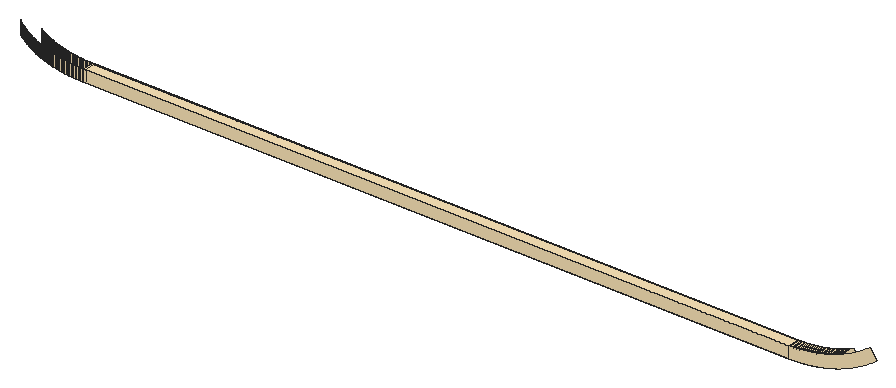
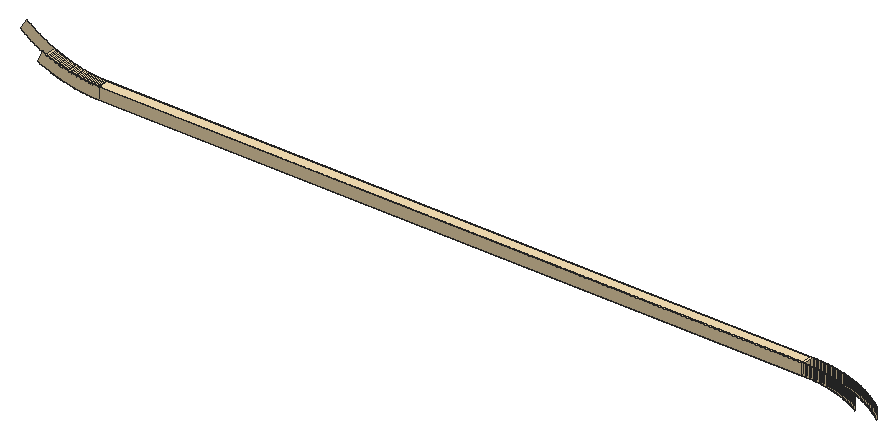
# SketchUp Ruby script. Lengths in inches.
U = 1.inch
M = Sketchup.active_model
def pt(a) = Geom::Point3d.new(a.map { |v| v * U })
def face(e, loops, mat)
  f = e.add_face(loops[0].map { |a| pt(a) })
  loops[1..].each { |l| e.add_face(l.map { |a| pt(a) }).erase! }
  f.material = f.back_material = mat if mat
  f
end
# faces: each face lists its corners as indices into pts; further lists are holes
def faces(e, pts, list, mat = nil) = list.each { |f| face(e, (f[0].is_a?(Array) ? f : [f]).map { |l| l.map { |i| pts[i] } }, mat) }
# xy, xz, yz: faces in a plane at the given z, y or x. An outline is a flat list of corners, or four numbers for a rectangle; further outlines are holes
def ring(l) = l.size == 4 ? [[l[0], l[1]], [l[2], l[1]], [l[2], l[3]], [l[0], l[3]]] : l.each_slice(2).to_a
def flat(e, list, mat, &to3) = list.each { |f| face(e, (f[0].is_a?(Array) ? f : [f]).map { |l| ring(l).map { |u, v| to3.(u, v) } }, mat) }
def xy(e, z, list, mat = nil) = flat(e, list, mat) { |x, y| [x, y, z] }
def xz(e, y, list, mat = nil) = flat(e, list, mat) { |x, z| [x, y, z] }
def yz(e, x, list, mat = nil) = flat(e, list, mat) { |y, z| [x, y, z] }
def lines(e, pts, list) = list.each { |a, b| e.add_line(pt(pts[a]), pt(pts[b])) }
# prism: a flat outline (further loops are holes) pulled along v
def prism(e, loops, v, mat = nil)
  f = face(e, loops, mat); d = Geom::Vector3d.new(v.map { |x| x * U })
  f.pushpull(f.normal.samedirection?(d) ? d.length : -d.length)
end
def box(e, o, s, mat = nil) = prism(e, [[o, [o[0] + s[0], o[1], o[2]], [o[0] + s[0], o[1] + s[1], o[2]], [o[0], o[1] + s[1], o[2]]]], [0, 0, s[2]], mat)
def at(x, y, z, deg = 0) = Geom::Transformation.translation(pt([x, y, z])) * Geom::Transformation.rotation(ORIGIN, Z_AXIS, deg.degrees)
def axes(o, x, y, z) = Geom::Transformation.new([*x, 0, *y, 0, *z, 0, *pt(o).to_a, 1])
def part(name) = M.definitions.add(name)
# library, detail: a bought-in or finely detailed component or shape, given as its bounding box
def library(name, o, s) = part(name).tap { |d| box(d.entities, o, s) }
def detail(e, o, s) = box(e.add_group.entities, o, s)
def put(e, d, t, mat = nil) = e.add_instance(d, t).tap { |i| i.material = mat if mat }
def group(e, t, mat = nil) = e.add_group.tap { |g| g.transformation = t; g.material = mat if mat }.entities
root = M.entities
M.materials.add("1026 AP 7946 SUNNY SIDE UP").color = [254, 231, 186]
xy(root,142,[[153.005,213.099,30,213.101,30,215.101,153.005,215.099],[29.752,213.101,29.765,215.001,29.766,215.101,30,215.101,30,213.101]],"1026 AP 7946 SUNNY SIDE UP")
xy(root,142.001,[[153.241,213.099,153.255,215.099]],"1026 AP 7946 SUNNY SIDE UP")
xy(root,144,[[153,213.099,153,215,30,215.001,30,215,30.001,213.101],[29.752,213.101,30.001,213.101,30,215,30,215.101,29.766,215.101,29.765,215.001],[153,215,153,215.099,30,215.101,30,215.001],[29.765,215.001,30,215.001,30,215.101,29.766,215.101]],"1026 AP 7946 SUNNY SIDE UP")
xy(root,144.001,[[153.231,213.099,153.236,215],[153.231,215,153.236,215.099]],"1026 AP 7946 SUNNY SIDE UP")
xz(root,213.099,[[153.005,142,153.241,142.001,153.255,142.001,153.51,142.005,153.766,142.011,154.021,142.02,154.276,142.031,154.531,142.045,154.785,142.061,155.04,142.08,155.294,142.101,155.548,142.125,155.802,142.151,156.056,142.18,156.309,142.211,156.5625,142.245,156.815,142.281,157.067,142.32,157.319,142.361,157.571,142.405,157.822,142.451,158.072,142.5,158.322,142.551,158.572,142.604,158.821,142.66,159.07,142.718,159.317,142.779,159.565,142.842,159.811,142.908,160.057,142.976,160.303,143.047,160.547,143.12,160.791,143.195,161.034,143.273,161.277,143.353,161.518,143.435,161.759,143.52,161.999,143.607,162.238,143.697,162.476,143.788,162.713,143.883,162.95,143.979,163.185,144.078,163.419,144.179,163.653,144.283,163.885,144.388,164.116,144.496,164.347,144.607,164.576,144.719,164.804,144.834,165.031,144.951,165.256,145.07,165.481,145.191,165.704,145.315,165.926,145.441,166.147,145.569,166.367,145.699,166.585,145.831,166.802,145.966,167.018,146.102,167.232,146.241,167.445,146.382,167.656,146.525,167.867,146.67,168.075,146.817,168.282,146.966,167.107,148.584,166.916,148.446,166.723,148.31,166.529,148.177,166.334,148.045,166.137,147.915,165.939,147.787,165.74,147.661,165.54,147.537,165.338,147.415,165.136,147.294,164.932,147.176,164.727,147.06,164.521,146.946,164.314,146.834,164.105,146.724,163.896,146.616,163.685,146.51,163.474,146.406,163.261,146.304,163.048,146.205,162.833,146.107,162.618,146.011,162.402,145.918,162.184,145.827,161.966,145.738,161.747,145.651,161.527,145.566,161.307,145.483,161.085,145.403,160.863,145.325,160.64,145.249,160.416,145.175,160.192,145.103,159.967,145.033,159.741,144.966,159.515,144.901,159.287,144.838,159.06,144.778,158.832,144.719,158.603,144.663,158.373,144.609,158.143,144.558,157.913,144.508,157.682,144.461,157.451,144.416,157.219,144.374,156.987,144.333,156.754,144.295,156.522,144.26,156.288,144.226,156.055,144.195,155.821,144.166,155.587,144.14,155.352,144.116,155.118,144.094,154.883,144.074,154.648,144.057,154.413,144.042,154.178,144.029,153.942,144.019,153.707,144.01,153.471,144.005,153.236,144.001,153.231,144.001,153,144]],"1026 AP 7946 SUNNY SIDE UP")
xz(root,213.101,[[29.752,142,30,142,30.001,144,29.752,144]],"1026 AP 7946 SUNNY SIDE UP")
xz(root,215.099,[[153.005,142,153,144,153.231,144.001,153.236,144.001,153.471,144.005,153.707,144.01,153.942,144.019,154.178,144.029,154.413,144.042,154.648,144.057,154.883,144.074,155.118,144.094,155.352,144.116,155.587,144.14,155.821,144.166,156.055,144.195,156.288,144.226,156.522,144.26,156.754,144.295,156.987,144.333,157.219,144.374,157.451,144.416,157.682,144.461,157.913,144.508,158.143,144.558,158.373,144.609,158.603,144.663,158.832,144.719,159.06,144.778,159.287,144.838,159.515,144.901,159.741,144.966,159.967,145.033,160.192,145.103,160.416,145.175,160.64,145.249,160.863,145.325,161.085,145.403,161.307,145.483,161.527,145.566,161.747,145.651,161.966,145.738,162.184,145.827,162.402,145.918,162.618,146.011,162.833,146.107,163.653,144.283,163.419,144.179,163.185,144.078,162.95,143.979,162.713,143.883,162.476,143.788,162.238,143.697,161.999,143.607,161.759,143.52,161.518,143.435,161.277,143.353,161.034,143.273,160.791,143.195,160.547,143.12,160.303,143.047,160.057,142.976,159.811,142.908,159.565,142.842,159.317,142.779,159.07,142.718,158.821,142.66,158.572,142.604,158.322,142.551,158.072,142.5,157.822,142.451,157.571,142.405,157.319,142.361,157.067,142.32,156.815,142.281,156.5625,142.245,156.309,142.211,156.056,142.18,155.802,142.151,155.548,142.125,155.294,142.101,155.04,142.08,154.785,142.061,154.531,142.045,154.276,142.031,154.021,142.02,153.766,142.011,153.51,142.005,153.255,142.001,153.241,142.001]],"1026 AP 7946 SUNNY SIDE UP")
xz(root,215.101,[[29.766,142,30,144]],"1026 AP 7946 SUNNY SIDE UP")
p = [[28.228,213.16,144],[28.228,213.16,142],[28.481,213.144,142],[28.481,213.144,144],[28.734,213.13,142],[28.734,213.13,144],
  [28.987,213.119,142],[28.987,213.119,144],[29.24,213.111,142],[29.24,213.111,144],[29.493,213.104,142],[29.493,213.104,144],
  [29.752,213.101,142],[29.752,213.101,144],[30.001,213.101,144],[30,213.101,142],[153.005,213.099,142],[153,213.099,144],
  [153.005,215.099,142],[153.241,215.099,142.001],[153.241,213.099,142.001],[153.255,213.099,142.001],[153.255,215.099,142.001],[153.51,215.099,142.005],
  [153.51,213.099,142.005],[153.766,215.099,142.011],[153.766,213.099,142.011],[154.021,215.099,142.02],[154.021,213.099,142.02],[154.276,215.099,142.031],
  [154.276,213.099,142.031],[154.531,215.099,142.045],[154.531,213.099,142.045],[154.785,215.099,142.061],[154.785,213.099,142.061],[26.967,213.278,144],
  [26.967,213.278,142],[27.218,213.25,142],[27.218,213.25,144],[27.47,213.224,142],[27.47,213.224,144],[27.723,213.2,142],
  [27.723,213.2,144],[27.975,213.179,142],[27.975,213.179,144],[26.213,213.378,144],[26.213,213.378,142],[26.464,213.342,142],
  [26.464,213.342,144],[26.715,213.309,142],[26.715,213.309,144],[25.713,213.458,144],[25.713,213.458,142],[25.963,213.417,142],
  [25.963,213.417,144],[24.965,213.595,144],[24.965,213.595,142],[25.214,213.547,142],[25.214,213.547,144],[25.463,213.501,142],
  [25.463,213.501,144],[24.469,213.698,144],[24.469,213.698,142],[24.717,213.645,142],[24.717,213.645,144],[24.222,213.754,144],
  [24.222,213.754,142],[23.729,213.872,144],[23.729,213.872,142],[23.975,213.812,142],[23.975,213.812,144],[23.239,214,144],
  [23.239,214,142],[23.484,213.935,142],[23.484,213.935,144],[22.994,214.067,144],[22.994,214.067,142],[22.508,214.209,144],
  [22.508,214.209,142],[22.751,214.137,142],[22.751,214.137,144],[22.266,214.284,144],[22.266,214.284,142],[22.025,214.361,144],
  [22.025,214.361,142],[21.544,214.522,144],[21.544,214.522,142],[21.784,214.44,142],[21.784,214.44,144],[21.305,214.606,144],
  [21.305,214.606,142],[21.067,214.693,144],[21.067,214.693,142],[20.83,214.781,144],[20.83,214.781,142],[20.593,214.872,144],
  [20.593,214.872,142],[20.358,214.966,144],[20.358,214.966,142],[20.123,215.062,144],[20.123,215.062,142],[19.889,215.16,144],
  [19.889,215.16,142],[28.365,215.156,142],[28.365,215.156,144],[28.598,215.141,144],[28.598,215.141,142],[28.832,215.128,144],
  [28.832,215.128,142],[29.065,215.118,144],[29.065,215.118,142],[29.299,215.11,144],[29.299,215.11,142],[29.533,215.104,144],
  [29.533,215.104,142],[29.766,215.101,144],[29.766,215.101,142],[30,215.101,142],[30,215.101,144],[153,215.099,144],
  [19.657,215.26,144],[19.657,215.26,142],[27.201,215.264,142],[27.201,215.264,144],[27.434,215.238,144],[27.434,215.238,142],
  [27.666,215.214,144],[27.666,215.214,142],[27.899,215.192,144],[27.899,215.192,142],[28.132,215.173,144],[28.132,215.173,142],
  [19.425,215.362,144],[19.425,215.362,142],[26.506,215.357,142],[26.506,215.357,144],[26.738,215.324,144],[26.738,215.324,142],
  [26.969,215.293,144],[26.969,215.293,142],[19.194,215.467,144],[19.194,215.467,142],[25.814,215.47,142],[25.814,215.47,144],
  [26.044,215.43,144],[26.044,215.43,142],[26.275,215.392,144],[26.275,215.392,142],[18.965,215.574,144],[18.965,215.574,142],
  [25.355,215.556,142],[25.355,215.556,144],[25.584,215.512,144],[25.584,215.512,142],[18.736,215.684,144],[18.736,215.684,142],
  [24.897,215.652,142],[24.897,215.652,144],[25.126,215.603,144],[25.126,215.603,142],[18.509,215.795,144],[18.509,215.795,142],
  [24.441,215.756,142],[24.441,215.756,144],[24.669,215.703,144],[24.669,215.703,142],[18.282,215.909,144],[18.282,215.909,142],
  [23.988,215.87,142],[23.988,215.87,144],[24.214,215.812,144],[24.214,215.812,142],[18.057,216.025,144],[18.057,216.025,142],
  [23.537,215.992,142],[23.537,215.992,144],[23.762,215.93,144],[23.762,215.93,142],[17.833,216.143,144],[17.833,216.143,142],
  [23.312,216.057,142],[23.312,216.057,144],[17.61,216.264,144],[17.61,216.264,142],[22.865,216.192,142],[22.865,216.192,144],
  [23.088,216.123,144],[23.088,216.123,142],[22.642,216.263,142],[22.642,216.263,144],[17.388,216.386,144],[17.388,216.386,142],
  [22.199,216.412,142],[22.199,216.412,144],[22.42,216.337,144],[22.42,216.337,142],[17.168,216.511,144],[17.168,216.511,142],
  [21.978,216.49,142],[21.978,216.49,144],[16.948,216.638,144],[16.948,216.638,142],[21.758,216.569,142],[21.758,216.569,144],
  [16.73,216.767,144],[16.73,216.767,142],[21.539,216.651,142],[21.539,216.651,144],[21.104,216.821,142],[21.104,216.821,144],
  [21.321,216.735,144],[21.321,216.735,142],[16.514,216.898,144],[16.514,216.898,142],[20.888,216.91,142],[20.888,216.91,144],
  [16.298,217.031,144],[16.298,217.031,142],[20.672,217,142],[20.672,217,144],[16.084,217.167,144],[16.084,217.167,142],
  [20.457,217.093,142],[20.457,217.093,144],[20.244,217.187,142],[20.244,217.187,144],[15.871,217.304,144],[15.871,217.304,142],
  [20.031,217.284,142],[20.031,217.284,144],[15.66,217.444,144],[15.66,217.444,142],[19.819,217.383,142],[19.819,217.383,144],
  [15.45,217.585,144],[15.45,217.585,142],[19.608,217.484,142],[19.608,217.484,144],[19.398,217.587,142],[19.398,217.587,144],
  [15.241,217.729,144],[15.241,217.729,142],[19.189,217.691,142],[19.189,217.691,144],[15.034,217.875,144],[15.034,217.875,142],
  [18.981,217.799,142],[18.981,217.799,144],[18.775,217.908,142],[18.775,217.908,144],[14.828,218.023,144],[14.828,218.023,142],
  [18.569,218.019,142],[18.569,218.019,144],[14.624,218.172,144],[14.624,218.172,142],[18.364,218.132,142],[18.364,218.132,144],
  [18.161,218.247,142],[18.161,218.247,144],[14.421,218.324,144],[14.421,218.324,142],[155.04,215.099,142.08],[155.04,213.099,142.08],
  [155.294,215.099,142.101],[155.294,213.099,142.101],[155.548,215.099,142.125],[155.548,213.099,142.125],[155.802,215.099,142.151],[155.802,213.099,142.151],
  [156.056,215.099,142.18],[156.056,213.099,142.18],[156.309,215.099,142.211],[156.309,213.099,142.211],[156.5625,215.099,142.245],[156.5625,213.099,142.245],
  [156.815,215.099,142.281],[156.815,213.099,142.281],[157.067,215.099,142.32],[157.067,213.099,142.32],[157.319,215.099,142.361],[157.319,213.099,142.361],
  [157.571,215.099,142.405],[157.571,213.099,142.405],[157.822,215.099,142.451],[157.822,213.099,142.451],[158.072,215.099,142.5],[158.072,213.099,142.5],
  [158.322,215.099,142.551],[158.322,213.099,142.551],[158.572,215.099,142.604],[158.572,213.099,142.604],[158.821,215.099,142.66],[158.821,213.099,142.66],
  [159.07,215.099,142.718],[159.07,213.099,142.718],[159.317,215.099,142.779],[159.317,213.099,142.779],[159.565,215.099,142.842],[159.565,213.099,142.842],
  [159.811,215.099,142.908],[159.811,213.099,142.908],[160.057,215.099,142.976],[160.057,213.099,142.976],[160.303,215.099,143.047],[160.303,213.099,143.047],
  [160.547,215.099,143.12],[160.547,213.099,143.12],[160.791,215.099,143.195],[160.791,213.099,143.195],[161.034,215.099,143.273],[161.034,213.099,143.273],
  [161.277,215.099,143.353],[161.277,213.099,143.353],[161.518,215.099,143.435],[161.518,213.099,143.435],[161.759,215.099,143.52],[161.759,213.099,143.52],
  [161.999,215.099,143.607],[161.999,213.099,143.607],[162.238,215.099,143.697],[162.238,213.099,143.697],[153.231,213.099,144.001],[153.231,215,144.001],
  [153,215,144],[153.471,213.099,144.005],[153.471,215,144.005],[153.236,215,144.001],[153.236,213.099,144.001],[153.707,213.099,144.01],
  [153.707,215,144.01],[153.942,213.099,144.019],[153.942,215,144.019],[154.178,213.099,144.029],[154.178,215,144.029],[154.413,213.099,144.042],
  [154.413,215,144.042],[154.648,213.099,144.057],[154.648,215,144.057],[153.231,215.099,144.001],[153.236,215.099,144.001],[153.471,215.099,144.005],
  [153.707,215.099,144.01],[153.942,215.099,144.019],[154.178,215.099,144.029],[154.413,215.099,144.042],[154.648,215.099,144.057],[154.883,213.099,144.074],
  [154.883,215,144.074],[155.118,213.099,144.094],[155.118,215,144.094],[155.352,213.099,144.116],[155.352,215,144.116],[155.587,213.099,144.14],
  [155.587,215,144.14],[155.821,213.099,144.166],[155.821,215,144.166],[154.883,215.099,144.074],[155.118,215.099,144.094],[155.352,215.099,144.116],
  [155.587,215.099,144.14],[155.821,215.099,144.166],[156.055,213.099,144.195],[156.055,215,144.195],[156.288,213.099,144.226],[156.288,215,144.226],
  [156.522,213.099,144.26],[156.522,215,144.26],[156.055,215.099,144.195],[156.288,215.099,144.226],[156.522,215.099,144.26],[156.754,213.099,144.295],
  [156.754,215,144.295],[156.987,213.099,144.333],[156.987,215,144.333],[157.219,213.099,144.374],[157.219,215,144.374],[156.754,215.099,144.295],
  [156.987,215.099,144.333],[157.219,215.099,144.374],[157.451,213.099,144.416],[157.451,215,144.416],[157.682,213.099,144.461],[157.682,215,144.461],
  [157.451,215.099,144.416],[157.682,215.099,144.461],[157.913,213.099,144.508],[157.913,215,144.508],[158.143,213.099,144.558],[158.143,215,144.558],
  [157.913,215.099,144.508],[158.143,215.099,144.558],[158.373,213.099,144.609],[158.373,215,144.609],[158.603,213.099,144.663],[158.603,215,144.663],
  [158.373,215.099,144.609],[158.603,215.099,144.663],[158.832,213.099,144.719],[158.832,215,144.719],[159.06,213.099,144.778],[159.06,215,144.778],
  [158.832,215.099,144.719],[159.06,215.099,144.778],[159.287,213.099,144.838],[159.287,215,144.838],[159.515,213.099,144.901],[159.515,215,144.901],
  [159.287,215.099,144.838],[159.515,215.099,144.901],[159.741,213.099,144.966],[159.741,215,144.966],[159.741,215.099,144.966],[159.967,213.099,145.033],
  [159.967,215,145.033],[160.192,213.099,145.103],[160.192,215,145.103],[159.967,215.099,145.033],[160.192,215.099,145.103],[160.416,213.099,145.175],
  [160.416,215,145.175],[160.416,215.099,145.175],[160.64,213.099,145.249],[160.64,215,145.249],[160.863,213.099,145.325],[160.863,215,145.325],
  [160.64,215.099,145.249],[160.863,215.099,145.325],[161.085,213.099,145.403],[161.085,215,145.403],[161.085,215.099,145.403],[161.307,213.099,145.483],
  [161.307,215,145.483],[161.307,215.099,145.483],[161.527,213.099,145.566],[161.527,215,145.566],[161.527,215.099,145.566],[161.747,213.099,145.651],
  [161.747,215,145.651],[161.747,215.099,145.651],[161.966,213.099,145.738],[161.966,215,145.738],[162.184,213.099,145.827],[162.184,215,145.827],
  [161.966,215.099,145.738],[162.184,215.099,145.827]]
faces(root,p,[[0,1,2,3],[3,2,4,5],[5,4,6,7],[7,6,8,9],[9,8,10,11],[11,10,12,13],[14,15,16,17],[16,18,19,20],
  [21,22,23,24],[24,23,25,26],[26,25,27,28],[28,27,29,30],[30,29,31,32],[32,31,33,34],[35,36,37,38],[38,37,39,40],
  [40,39,41,42],[42,41,43,44],[44,43,1,0],[45,46,47,48],[48,47,49,50],[50,49,36,35],[51,52,53,54],[54,53,46,45],
  [55,56,57,58],[58,57,59,60],[60,59,52,51],[61,62,63,64],[64,63,56,55],[65,66,62,61],[67,68,69,70],[70,69,66,65],
  [71,72,73,74],[74,73,68,67],[75,76,72,71],[77,78,79,80],[80,79,76,75],[81,82,78,77],[83,84,82,81],[85,86,87,88],
  [88,87,84,83],[89,90,86,85],[91,92,90,89],[93,94,92,91],[95,96,94,93],[97,98,96,95],[99,100,98,97],[101,102,100,99],
  [103,104,105,106],[106,105,107,108],[108,107,109,110],[110,109,111,112],[112,111,113,114],[114,113,115,116],[117,118,119,18],[120,121,102,101],
  [122,123,124,125],[125,124,126,127],[127,126,128,129],[129,128,130,131],[131,130,104,103],[132,133,121,120],[134,135,136,137],[137,136,138,139],
  [139,138,123,122],[140,141,133,132],[142,143,144,145],[145,144,146,147],[147,146,135,134],[148,149,141,140],[150,151,152,153],[153,152,143,142],
  [154,155,149,148],[156,157,158,159],[159,158,151,150],[160,161,155,154],[162,163,164,165],[165,164,157,156],[166,167,161,160],[168,169,170,171],
  [171,170,163,162],[172,173,167,166],[174,175,176,177],[177,176,169,168],[178,179,173,172],[180,181,175,174],[182,183,179,178],[184,185,186,187],
  [187,186,181,180],[188,189,185,184],[190,191,183,182],[192,193,194,195],[195,194,189,188],[196,197,191,190],[198,199,193,192],[200,201,197,196],
  [202,203,199,198],[204,205,201,200],[206,207,203,202],[208,209,210,211],[211,210,207,206],[212,213,205,204],[214,215,209,208],[216,217,213,212],
  [218,219,215,214],[220,221,217,216],[222,223,219,218],[224,225,223,222],[226,227,221,220],[228,229,225,224],[230,231,227,226],[232,233,229,228],
  [234,235,231,230],[236,237,233,232],[238,239,237,236],[240,241,235,234],[242,243,239,238],[244,245,241,240],[246,247,243,242],[248,249,247,246],
  [250,251,245,244],[252,253,249,248],[254,255,251,250],[256,257,253,252],[258,259,257,256],[260,261,255,254],[34,33,262,263],[263,262,264,265],
  [265,264,266,267],[267,266,268,269],[269,268,270,271],[271,270,272,273],[273,272,274,275],[275,274,276,277],[277,276,278,279],[279,278,280,281],
  [281,280,282,283],[283,282,284,285],[285,284,286,287],[287,286,288,289],[289,288,290,291],[291,290,292,293],[293,292,294,295],[295,294,296,297],
  [297,296,298,299],[299,298,300,301],[301,300,302,303],[303,302,304,305],[305,304,306,307],[307,306,308,309],[309,308,310,311],[311,310,312,313],
  [313,312,314,315],[315,314,316,317],[317,316,318,319],[319,318,320,321],[322,323,324,17],[325,326,327,328],[329,330,326,325],[331,332,330,329],
  [333,334,332,331],[335,336,334,333],[337,338,336,335],[119,324,323,339],[340,327,326,341],[341,326,330,342],[342,330,332,343],[343,332,334,344],
  [344,334,336,345],[345,336,338,346],[347,348,338,337],[349,350,348,347],[351,352,350,349],[353,354,352,351],[355,356,354,353],[346,338,348,357],
  [357,348,350,358],[358,350,352,359],[359,352,354,360],[360,354,356,361],[362,363,356,355],[364,365,363,362],[366,367,365,364],[361,356,363,368],
  [368,363,365,369],[369,365,367,370],[371,372,367,366],[373,374,372,371],[375,376,374,373],[370,367,372,377],[377,372,374,378],[378,374,376,379],
  [380,381,376,375],[382,383,381,380],[379,376,381,384],[384,381,383,385],[386,387,383,382],[388,389,387,386],[385,383,387,390],[390,387,389,391],
  [392,393,389,388],[394,395,393,392],[391,389,393,396],[396,393,395,397],[398,399,395,394],[400,401,399,398],[397,395,399,402],[402,399,401,403],
  [404,405,401,400],[406,407,405,404],[403,401,405,408],[408,405,407,409],[410,411,407,406],[409,407,411,412],[413,414,411,410],[415,416,414,413],
  [412,411,414,417],[417,414,416,418],[419,420,416,415],[418,416,420,421],[422,423,420,419],[424,425,423,422],[421,420,423,426],[426,423,425,427],
  [428,429,425,424],[427,425,429,430],[431,432,429,428],[430,429,432,433],[434,435,432,431],[433,432,435,436],[437,438,435,434],[436,435,438,439],
  [440,441,438,437],[442,443,441,440],[439,438,441,444],[444,441,443,445]],"1026 AP 7946 SUNNY SIDE UP")
